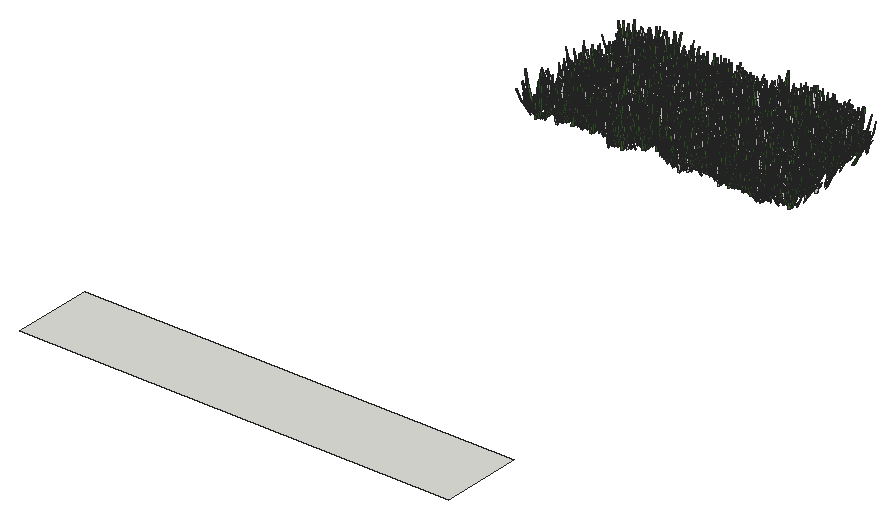
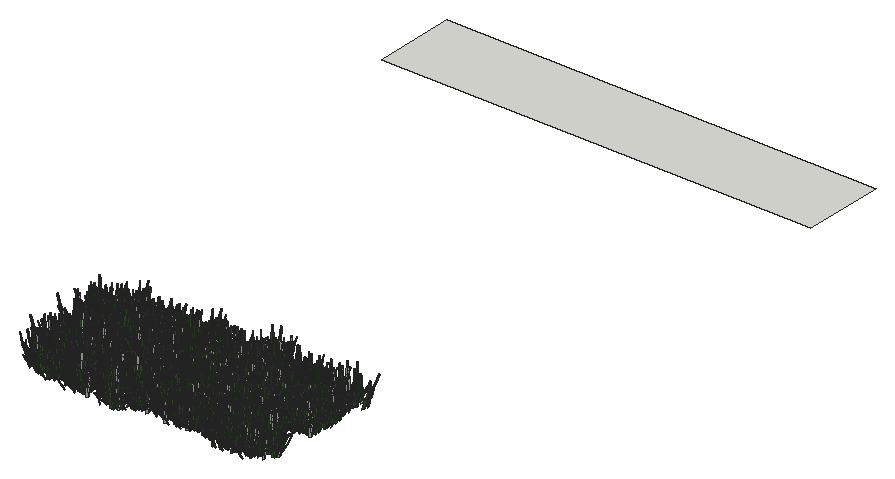
# SketchUp Ruby script. Lengths in inches.
U = 1.inch
M = Sketchup.active_model
def pt(a) = Geom::Point3d.new(a.map { |v| v * U })
def face(e, loops, mat)
  f = e.add_face(loops[0].map { |a| pt(a) })
  loops[1..].each { |l| e.add_face(l.map { |a| pt(a) }).erase! }
  f.material = f.back_material = mat if mat
  f
end
# faces: each face lists its corners as indices into pts; further lists are holes
def faces(e, pts, list, mat = nil) = list.each { |f| face(e, (f[0].is_a?(Array) ? f : [f]).map { |l| l.map { |i| pts[i] } }, mat) }
# xy, xz, yz: faces in a plane at the given z, y or x. An outline is a flat list of corners, or four numbers for a rectangle; further outlines are holes
def ring(l) = l.size == 4 ? [[l[0], l[1]], [l[2], l[1]], [l[2], l[3]], [l[0], l[3]]] : l.each_slice(2).to_a
def flat(e, list, mat, &to3) = list.each { |f| face(e, (f[0].is_a?(Array) ? f : [f]).map { |l| ring(l).map { |u, v| to3.(u, v) } }, mat) }
def xy(e, z, list, mat = nil) = flat(e, list, mat) { |x, y| [x, y, z] }
def xz(e, y, list, mat = nil) = flat(e, list, mat) { |x, z| [x, y, z] }
def yz(e, x, list, mat = nil) = flat(e, list, mat) { |y, z| [x, y, z] }
def lines(e, pts, list) = list.each { |a, b| e.add_line(pt(pts[a]), pt(pts[b])) }
# prism: a flat outline (further loops are holes) pulled along v
def prism(e, loops, v, mat = nil)
  f = face(e, loops, mat); d = Geom::Vector3d.new(v.map { |x| x * U })
  f.pushpull(f.normal.samedirection?(d) ? d.length : -d.length)
end
def box(e, o, s, mat = nil) = prism(e, [[o, [o[0] + s[0], o[1], o[2]], [o[0] + s[0], o[1] + s[1], o[2]], [o[0], o[1] + s[1], o[2]]]], [0, 0, s[2]], mat)
def at(x, y, z, deg = 0) = Geom::Transformation.translation(pt([x, y, z])) * Geom::Transformation.rotation(ORIGIN, Z_AXIS, deg.degrees)
def axes(o, x, y, z) = Geom::Transformation.new([*x, 0, *y, 0, *z, 0, *pt(o).to_a, 1])
def part(name) = M.definitions.add(name)
# library, detail: a bought-in or finely detailed component or shape, given as its bounding box
def library(name, o, s) = part(name).tap { |d| box(d.entities, o, s) }
def detail(e, o, s) = box(e.add_group.entities, o, s)
def put(e, d, t, mat = nil) = e.add_instance(d, t).tap { |i| i.material = mat if mat }
def group(e, t, mat = nil) = e.add_group.tap { |g| g.transformation = t; g.material = mat if mat }.entities
root = M.entities
M.materials.add("Material1").color = [58, 110, 58]
M.materials.add("Material10").color = [48, 100, 38]
M.materials.add("Material3").color = [68, 110, 58]
M.materials.add("Material4").color = [48, 90, 38]
M.materials.add("Material5").color = [68, 110, 48]
M.materials.add("Material6").color = [48, 90, 48]
M.materials.add("Material8").color = [58, 90, 38]
M.materials.add("Material9").color = [68, 100, 58]
c1 = part("grass00")
p = [[-0.6875,0.15,0],[-0.56,0.08,5.52],[-0.04,0.03,2.76],[0.48,-0.02,0],[0.35,-0.02,5.52],[-0.1,-0.14,5.52],
  [-0.12,0.65,8.37],[-0.42,0.65,8.37]]
faces(c1.entities,p,[[0,1,2,3],[3,2,4],[1,5,2],[5,4,2],[1,6,5],[4,5,6],[7,6,1]])
c2 = part("Group16\#1")
put(c2.entities,c1,axes([1.44,-0.61,-0.01],[0.05352,0.12609,0],[-0.10704,0.04543,0.07239],[0.06664,-0.02828,0.11628]),"Material6")
put(c2.entities,c1,axes([0.76,-0.15,-0.01],[0.04676,0.24062,0],[-0.23162,0.04501,0.06642],[0.0652,-0.01267,0.23595]),"Material3")
put(c2.entities,c1,axes([0.79,0.01,-0.01],[-0.00606,0.34651,0],[-0.34381,-0.00602,0.0432],[0.04319,0.00076,0.34386]))
put(c2.entities,c1,axes([1,0.23,-0.01],[-0.07192,0.31144,0],[-0.28722,-0.06632,0.1236],[0.12043,0.02781,0.29478]),"Material5")
put(c2.entities,c1,axes([1.66,0.77,-0.01],[-0.13828,0.29651,0],[-0.21551,-0.1005,0.22471],[0.20365,0.09498,0.23779]),"Material10")
put(c2.entities,c1,axes([0.6875,0.52,-0.01],[-0.18126,0.24051,0],[-0.22746,-0.17142,0.09788],[0.07817,0.05891,0.28481]),"Material5")
put(c2.entities,c1,axes([0.68,0.78,-0.01],[-0.215,0.18688,0],[-0.12385,-0.14248,0.21334],[0.13995,0.16101,0.18878]),"Material3")
put(c2.entities,c1,axes([0.56,1,-0.01],[-0.13756,0.07624,0],[-0.06159,-0.11112,0.0927],[0.04494,0.08108,0.12705]),"Material5")
put(c2.entities,c1,axes([0.2,0.64,-0.01],[-0.23729,0.07254,0],[-0.05711,-0.18681,0.153],[0.04473,0.14632,0.19535]),"Material10")
put(c2.entities,c1,axes([0.0625,0.72,-0.01],[-0.28874,0.02525,0],[-0.02179,-0.24916,0.14647],[0.01276,0.14591,0.25012]),"Material3")
put(c2.entities,c1,axes([-0.08,0.62,-0.01],[-0.34089,-0.04187,0],[0.03255,-0.26504,0.216],[-0.02633,0.21439,0.26703]),"Material10")
put(c2.entities,c1,axes([-0.34,0.98,-0.01],[-0.14314,-0.0493,0],[0.04397,-0.12769,0.06843],[-0.02228,0.0647,0.13505]),"Material10")
put(c2.entities,c1,axes([-0.87,1.45,-0.01],[-0.23488,-0.14114,0],[0.13761,-0.22901,0.06087],[-0.03135,0.05217,0.26717]))
put(c2.entities,c1,axes([-0.72,0.77,-0.01],[-0.14208,-0.13251,0],[0.07209,-0.0773,0.16301],[-0.11118,0.11922,0.1057]),"Material10")
put(c2.entities,c1,axes([-0.62,0.43,-0.01],[-0.14845,-0.21203,0],[0.18654,-0.13061,0.12304],[-0.10079,0.07057,0.22772]),"Material3")
put(c2.entities,c1,axes([-0.68,0.29,-0.01],[-0.13639,-0.32136,0],[0.31723,-0.13464,0.05579],[-0.05136,0.0218,0.34462]),"Material4")
put(c2.entities,c1,axes([-0.64,0.125,-0.01],[-0.0458,-0.23569,0],[0.22124,-0.043,0.08276],[-0.08124,0.01579,0.22538]),"Material1")
put(c2.entities,c1,axes([-1.6,-0.03,-0.01],[0.00576,-0.32897,0],[0.27526,0.00482,0.18018],[-0.18015,-0.00315,0.2753]),"Material5")
put(c2.entities,c1,axes([-1.36,-0.31,-0.01],[0.05718,-0.24765,0],[0.18172,0.04196,0.17267],[-0.16825,-0.03885,0.1865]),"Material10")
put(c2.entities,c1,axes([-1.54,-0.72,-0.01],[0.06537,-0.14017,0],[0.13555,0.06321,0.03939],[-0.0357,-0.01665,0.14956]))
put(c2.entities,c1,axes([-1.19,-0.9,-0.01],[0.09597,-0.12735,0],[0.11214,0.08451,0.07557],[-0.06035,-0.04548,0.14042]),"Material9")
put(c2.entities,c1,axes([-0.47,-0.54,-0.01],[0.11588,-0.10072,0],[0.0618,0.0711,0.12124],[-0.07953,-0.0915,0.0942]))
put(c2.entities,c1,axes([-0.47,-0.84,-0.01],[0.11927,-0.0661,0],[0.06603,0.11913,0.00646],[-0.00313,-0.00565,0.13621]),"Material5")
put(c2.entities,c1,axes([-0.38,-1.24,-0.01],[0.28037,-0.08571,0],[0.0618,0.20215,0.20315],[-0.05939,-0.19428,0.21139]),"Material9")
put(c2.entities,c1,axes([-0.06,-0.66,-0.01],[0.22719,-0.01987,0],[0.01247,0.14255,0.17758],[-0.01547,-0.17691,0.1431]),"Material8")
put(c2.entities,c1,axes([0.11,-0.89,-0.01],[0.14882,0.01828,0],[-0.01058,0.08611,0.12229],[0.01491,-0.12138,0.08676]),"Material6")
put(c2.entities,c1,axes([0.25,-0.72,-0.01],[0.20481,0.07053,0],[-0.06206,0.18022,0.10291],[0.03351,-0.0973,0.1906]),"Material6")
put(c2.entities,c1,axes([0.85,-1.42,-0.01],[0.16481,0.09904,0],[-0.09472,0.15762,0.05616],[0.02893,-0.04814,0.18389]),"Material5")
put(c2.entities,c1,axes([1.01,-1.09,-0.01],[0.21858,0.20385,0],[-0.17495,0.1876,0.15339],[0.10462,-0.11218,0.25652]),"Material10")
put(c2.entities,c1,axes([1.01,-0.71,-0.01],[0.08733,0.12473,0],[-0.06445,0.04512,0.13037],[0.1068,-0.07477,0.07867]),"Material6")
c3 = part("Group15\#1")
put(c3.entities,c2,at(0,0,0))
c4 = part("3darcstudiotree_grass00\#1")
put(c4.entities,c3,at(0,0,0))
xy(root,0,[[282.38,19.38,346,31.39]])
put(root,c4,axes([297.61,97.11,0.25],[1.11442,-0.27325,0],[0.34617,0.97258,-0.05518],[0.02268,0.06373,1.77288]))
put(root,c4,axes([309.04,97.14,0.25],[-0.81622,0.63511,0],[-0.72135,-0.63864,-0.04557],[-0.05793,-0.05129,1.96028]))
put(root,c4,axes([318.15,97.38,0.25],[-0.95081,0.11233,0],[-0.13919,-0.81164,-0.03826],[-0.00903,-0.05267,1.65468]))
put(root,c4,axes([324.87,97.82,0.25],[0.99592,-0.02661,0],[0.02899,0.74764,-0.04101],[0.00201,0.05178,1.37186]))
put(root,c4,axes([326.48,98.03,0.25],[1.16611,0.10212,0],[-0.10117,0.79586,-0.03171],[-0.00592,0.04657,1.71518]))
put(root,c4,axes([330.21,97.79,0.25],[0.11865,0.89123,0],[-0.92054,0.08443,-0.03685],[-0.06873,0.0063,1.73767]))
put(root,c4,axes([304.1,98.11,0.25],[1.12096,0.07204,0],[-0.08662,0.92856,-0.0417],[-0.00549,0.05888,1.91485]))
put(root,c4,axes([324.01,97.96,0.25],[-0.93317,0.25697,0],[-0.32463,-0.81214,-0.04681],[-0.02202,-0.05508,1.53984]))
put(root,c4,axes([300.77,97.91,0.25],[-0.99958,0.5509,0],[-0.69845,-0.87305,-0.05111],[-0.03443,-0.04304,1.53759]))
put(root,c4,axes([308.39,98.12,0.25],[-0.94502,0.15563,0],[-0.24855,-1.03972,-0.05548],[-0.01391,-0.05818,1.6451]))
put(root,c4,axes([302.0625,98.48,0.25],[0.91722,-0.25224,0],[0.3035,0.7603,-0.03222],[0.01878,0.04704,1.78787]))
put(root,c4,axes([332.7,98.4375,0.25],[1.19981,0.30777,0],[-0.3695,0.99233,-0.04987],[-0.01901,0.05104,1.61513]))
put(root,c4,axes([328.71,98.2,0.25],[-0.13885,0.83735,0],[-1.13883,-0.13009,-0.0385],[-0.05163,-0.0059,1.55608]))
put(root,c4,axes([318.98,98.26,0.25],[0.07462,0.91972,0],[-0.97751,0.05464,-0.04154],[-0.07881,0.00441,1.86323]))
put(root,c4,axes([315.89,98.68,0.25],[0.09651,-0.80548,0],[0.96144,0.07936,-0.03727],[0.06649,0.00549,1.73202]))
put(root,c4,axes([321.23,98.59,0.25],[-0.42768,-0.67094,0],[0.95175,-0.41794,-0.0302],[0.04153,-0.01824,1.67548]))
put(root,c4,axes([311.67,98.66,0.25],[0.80756,0.80599,0],[-0.89495,0.61773,-0.02991],[-0.03862,0.02666,1.95467]))
put(root,c4,axes([322.41,99.12,0.25],[0.43279,-0.82555,0],[1.00075,0.36142,-0.04597],[0.05367,0.01938,1.38947]))
put(root,c4,axes([328.51,99.08,0.25],[-0.59328,0.73911,0],[-0.83118,-0.45962,-0.03773],[-0.04449,-0.0246,1.41517]))
put(root,c4,axes([299.35,99.12,0.25],[-0.22047,0.82927,0],[-1.14406,-0.20954,-0.05256],[-0.05732,-0.0105,1.30827]))
put(root,c4,axes([308.98,99.51,0.25],[0.31203,-0.81509,0],[1.23306,0.32518,-0.03698],[0.04985,0.01315,1.82987]))
put(root,c4,axes([317.5,99.3,0.25],[-1.00537,-0.3617,0],[0.36325,-0.69557,-0.04544],[0.0295,-0.05648,1.4908]))
put(root,c4,axes([304.08,99.45,0.25],[0.99013,0.44406,0],[-0.59296,0.91082,-0.05913],[-0.03144,0.0483,1.39517]))
put(root,c4,axes([324.36,99.86,0.25],[-0.68424,-0.62612,0],[0.77326,-0.58215,-0.0539],[0.05475,-0.04122,1.43163]))
put(root,c4,axes([312.68,99.88,0.25],[0.97858,0.24585,0],[-0.28536,0.7825,-0.0422],[-0.02332,0.06396,1.87907]))
put(root,c4,axes([301.36,99.81,0.25],[0.11207,0.80416,0],[-0.996,0.09562,-0.04522],[-0.0721,0.00692,1.60941]))
put(root,c4,axes([330.24,99.96,0.25],[-0.79621,-0.4404,0],[0.66053,-0.82267,-0.04785],[0.04066,-0.05064,1.82518]))
put(root,c4,axes([298.22,100.3125,0.25],[0.22875,-0.9605,0],[1.22208,0.2005,-0.04547],[0.0618,0.01014,1.72572]))
put(root,c4,axes([320.22,100.33,0.25],[1.29123,-0.11334,0],[0.13389,1.05087,-0.02611],[0.00423,0.03321,1.96192]))
put(root,c4,axes([313.45,100.29,0.25],[-0.17956,-0.84679,0],[1.25977,-0.18403,-0.05842],[0.08919,-0.01303,1.98292]))
put(root,c4,axes([302.2,100.43,0.25],[0.02759,0.77056,0],[-1.10892,0.02736,-0.05613],[-0.07716,0.0019,1.5259]))
put(root,c4,axes([331.22,100.58,0.25],[-0.75484,-0.55993,0],[0.64882,-0.60256,-0.04195],[0.04472,-0.04153,1.55746]))
put(root,c4,axes([318.8,100.71,0.25],[1.03911,0.09401,0],[-0.10137,0.77188,-0.03498],[-0.00601,0.0458,1.48455]))
put(root,c4,axes([324.91,100.49,0.25],[-0.85951,0.28596,0],[-0.412,-0.8531,-0.04281],[-0.0261,-0.05404,1.81418]))
put(root,c4,axes([314.73,100.51,0.25],[-0.22146,0.9116,0],[-1.23324,-0.20639,-0.03197],[-0.04449,-0.00745,1.78572]))
put(root,c4,axes([328.82,100.9,0.25],[1.17011,-0.34767,0],[0.39668,0.91972,-0.05713],[0.02422,0.05616,1.48067]))
put(root,c4,axes([311.82,100.56,0.25],[-0.5993,0.62128,0],[-0.79962,-0.53137,-0.02462],[-0.03671,-0.02439,1.95656]))
put(root,c4,axes([307.43,100.74,0.25],[0.05722,0.94648,0],[-1.16997,0.04872,-0.03261],[-0.05169,0.00215,1.85888]))
put(root,c4,axes([332.53,100.92,0.25],[-0.75241,-0.52207,0],[0.686,-0.6811,-0.04185],[0.04373,-0.04342,1.7425]))
put(root,c4,axes([304.37,100.9,0.25],[-1.04972,-0.29462,0],[0.37971,-0.93199,-0.06149],[0.02998,-0.07358,1.80385]))
put(root,c4,axes([310.51,101.17,0.25],[0.10575,-0.82311,0],[0.95887,0.08487,-0.04937],[0.08765,0.00776,1.72169]))
put(root,c4,axes([317.53,101.08,0.25],[0.831,0.29847,0],[-0.361,0.69242,-0.02703],[-0.02268,0.04351,1.9211]))
put(root,c4,axes([299.71,100.85,0.25],[-0.333,0.90097,0],[-0.9209,-0.23448,-0.03727],[-0.05842,-0.01487,1.57911]))
put(root,c4,axes([322.65,101.03,0.25],[-1.17026,-0.36941,0],[0.34854,-0.76064,-0.04106],[0.0256,-0.05587,1.71966]))
put(root,c4,axes([305.88,100.9,0.25],[-0.57732,0.57346,0],[-0.80073,-0.55534,-0.03387],[-0.03843,-0.02665,1.54303]))
put(root,c4,axes([309.86,101.96,0.25],[1.05783,0.04505,0],[-0.06563,1.06167,-0.05168],[-0.00349,0.05647,1.68853]))
put(root,c4,axes([297.7,101.96,0.25],[-0.14741,-0.93143,0],[0.95379,-0.10399,-0.04534],[0.07585,-0.00827,1.62314]))
put(root,c4,axes([323.3125,101.95,0.25],[-0.30211,-0.82943,0],[1.20998,-0.30361,-0.03772],[0.03909,-0.00981,1.36861]))
put(root,c4,axes([305.84,102.15,0.25],[0.91341,-0.33571,0],[0.50825,0.95265,-0.04981],[0.02823,0.05291,1.75709]))
put(root,c4,axes([326.74,101.86,0.25],[-1.11386,0.29268,0],[-0.32243,-0.84536,-0.03323],[-0.01665,-0.04365,1.77353]))
put(root,c4,axes([330.87,102.33,0.25],[1.03086,-0.47818,0],[0.57832,0.85889,-0.04605],[0.0263,0.03906,1.38783]))
put(root,c4,axes([315.96,101.99,0.25],[-0.9413,0.11811,0],[-0.18993,-1.04277,-0.03474],[-0.00584,-0.03204,1.42794]))
put(root,c4,axes([299.58,102.47,0.25],[0.63325,-0.82651,0],[0.82121,0.43345,-0.04064],[0.05169,0.02728,1.46692]))
put(root,c4,axes([329.73,102.18,0.25],[-0.64705,0.66274,0],[-0.92031,-0.61899,-0.04128],[-0.04141,-0.02785,1.52936]))
put(root,c4,axes([321.76,102.83,0.25],[1.05012,0.46296,0],[-0.47019,0.73472,-0.04207],[-0.03729,0.05828,1.89419]))
put(root,c4,axes([317.68,102.97,0.25],[-0.58739,0.78346,0],[-1.04255,-0.53848,-0.04897],[-0.06631,-0.03425,1.9584]))
put(root,c4,axes([316.28,103.14,0.25],[0.67846,0.67759,0],[-0.85974,0.59303,-0.05468],[-0.0598,0.04125,1.58958]))
put(root,c4,axes([306.8,103.52,0.25],[0.95094,-0.43354,0],[0.56411,0.8524,-0.02691],[0.01977,0.02987,1.78778]))
put(root,c4,axes([297.72,103.32,0.25],[-0.9964,-0.33803,0],[0.35737,-0.72569,-0.04864],[0.0279,-0.05665,1.4319]))
put(root,c4,axes([332.73,103.31,0.25],[-1.12743,-0.30714,0],[0.33973,-0.85911,-0.0393],[0.01924,-0.04865,1.71017]))
put(root,c4,axes([320.33,103.1875,0.25],[-0.89951,0.48737,0],[-0.66735,-0.8485,-0.04574],[-0.03789,-0.04818,1.85022]))
put(root,c4,axes([305.19,103.68,0.25],[0.59611,-0.65972,0],[0.97376,0.60614,-0.03529],[0.03147,0.01959,1.35654]))
put(root,c4,axes([310.63,103.33,0.25],[0.11273,0.93049,0],[-0.9606,0.08017,-0.04963],[-0.07565,0.00631,1.47912]))
put(root,c4,axes([326.61,104.0625,0.25],[-0.46457,-0.99645,0],[1.15948,-0.3724,-0.05475],[0.07745,-0.02488,1.88574]))
put(root,c4,axes([312.78,104.58,0.25],[0.42125,-0.83748,0],[1.16384,0.40329,-0.03949],[0.05184,0.01796,1.7941]))
put(root,c4,axes([328.78,104.7,0.25],[0.63809,-0.69669,0],[1.02647,0.64766,-0.05929],[0.05496,0.03468,1.50135]))
put(root,c4,axes([325.85,104.61,0.25],[-0.57071,-0.88679,0],[1.05327,-0.46697,-0.05822],[0.083,-0.0368,1.92982]))
put(root,c4,axes([329.61,104.72,0.25],[1.1093,0.03312,0],[-0.04015,0.92644,-0.02702],[-0.00174,0.04004,1.99535]))
put(root,c4,axes([310.17,104.7,0.25],[-0.85657,-0.75846,0],[0.78932,-0.61411,-0.03051],[0.03395,-0.02642,1.65027]))
put(root,c4,axes([320.77,104.93,0.25],[-0.86,-0.30499,0],[0.49403,-0.95969,-0.04539],[0.0273,-0.05303,1.92461]))
put(root,c4,axes([298.375,104.8125,0.25],[-0.66373,0.7804,0],[-0.8847,-0.51835,-0.04566],[-0.05684,-0.03331,1.65042]))
put(root,c4,axes([307.43,104.95,0.25],[-0.81395,0.35466,0],[-0.55874,-0.88338,-0.02543],[-0.01877,-0.02968,1.9093]))
put(root,c4,axes([325.57,105.72,0.25],[1.07758,0.21503,0],[-0.30245,1.04413,-0.03506],[-0.00839,0.02898,1.32515]))
put(root,c4,axes([297.92,105.64,0.25],[0.96578,0.31729,0],[-0.34767,0.72902,-0.04887],[-0.03524,0.07388,1.85053]))
put(root,c4,axes([300.12,106.1,0.25],[0.88355,-0.55441,0],[0.65814,0.72256,-0.04167],[0.04286,0.04705,1.86151]))
put(root,c4,axes([312.65,106.09,0.25],[0.37476,-0.82487,0],[1.09143,0.3416,-0.04892],[0.07598,0.02378,1.93615]))
put(root,c4,axes([311.34,105.75,0.25],[-1.08648,0.48141,0],[-0.55382,-0.86106,-0.03463],[-0.0258,-0.04011,1.86049]))
put(root,c4,axes([301.49,105.85,0.25],[0.38225,0.93797,0],[-0.99384,0.27902,-0.04556],[-0.06331,0.01777,1.53888]))
put(root,c4,axes([305.43,105.83,0.25],[-1.09946,0.15846,0],[-0.20428,-0.97645,-0.05401],[-0.01022,-0.04885,1.3206]))
put(root,c4,axes([314.78,105.86,0.25],[-0.84958,0.7153,0],[-0.71377,-0.58402,-0.05097],[-0.06552,-0.05361,1.80901]))
put(root,c4,axes([323.95,106.21,0.25],[0.95429,0.31987,0],[-0.42632,0.8762,-0.03343],[-0.02074,0.04263,1.88641]))
put(root,c4,axes([307.34,106.1,0.25],[0.55377,0.81028,0],[-0.78931,0.37162,-0.03898],[-0.07426,0.03496,1.98748]))
put(root,c4,axes([322.34,106.65,0.25],[0.24209,-0.99141,0],[1.19956,0.20179,-0.041],[0.05797,0.00975,1.76588]))
put(root,c4,axes([314.92,106.6,0.25],[1.2191,0.02658,0],[-0.027,0.85312,-0.04419],[-0.00224,0.07077,1.98467]))
put(root,c4,axes([311.93,106.71,0.25],[-0.47441,-0.8123,0],[0.87704,-0.35287,-0.03263],[0.05634,-0.02267,1.87]))
put(root,c4,axes([320.57,107.07,0.25],[1.2067,-0.00105,0],[0.00128,1.01679,-0.04894],[0.00006,0.04681,1.41164]))
put(root,c4,axes([331.68,107.02,0.25],[0.99274,0.22293,0],[-0.25761,0.79027,-0.04799],[-0.02037,0.0625,1.60328]))
put(root,c4,axes([313.64,107.03,0.25],[-0.97842,-0.39566,0],[0.51576,-0.87863,-0.02869],[0.02026,-0.03451,1.89824]))
put(root,c4,axes([323.66,107.1,0.25],[0.80414,0.72555,0],[-0.85103,0.64979,-0.033],[-0.03942,0.0301,1.87715]))
put(root,c4,axes([303.6,107,0.25],[-0.75001,0.80323,0],[-1.01098,-0.65032,-0.03455],[-0.03376,-0.02172,1.58129]))
put(root,c4,axes([315.7,107.18,0.25],[-0.02112,0.92901,0],[-1.11715,-0.0175,-0.05443],[-0.07643,-0.0012,1.56933]))
put(root,c4,axes([327.87,107.3125,0.25],[-1.1857,0.2388,0],[-0.30456,-1.04174,-0.06662],[-0.01699,-0.0581,1.39642]))
put(root,c4,axes([310.27,107.51,0.25],[-0.87437,0.41705,0],[-0.6352,-0.91743,-0.04948],[-0.03099,-0.04476,1.60238]))
put(root,c4,axes([324.25,108.01,0.25],[-0.31424,-0.81036,0],[1.12057,-0.29935,-0.0477],[0.05342,-0.01427,1.385]))
put(root,c4,axes([318.85,107.99,0.25],[-1.13196,0.07822,0],[-0.0777,-0.77461,-0.02559],[-0.00443,-0.04414,1.95328]))
put(root,c4,axes([317.96,107.96,0.25],[-0.77412,0.64338,0],[-0.79625,-0.65999,-0.05526],[-0.05902,-0.04892,1.69871]))
put(root,c4,axes([314.45,108.38,0.25],[-0.14115,-0.84151,0],[1.08164,-0.12498,-0.04493],[0.07806,-0.00902,1.91565]))
put(root,c4,axes([325.47,108.53,0.25],[0.45572,-0.66105,0],[0.90705,0.43077,-0.04415],[0.07294,0.03464,1.98924]))
put(root,c4,axes([327.2,108.64,0.25],[1.09438,-0.24928,0],[0.33452,1.01172,-0.05143],[0.01553,0.04697,1.44218]))
put(root,c4,axes([328.73,108.71,0.25],[0.53158,-0.96832,0],[1.00993,0.38194,-0.02827],[0.04498,0.01701,1.94019]))
put(root,c4,axes([321.96,108.36,0.25],[0.25266,1.02917,0],[-1.10373,0.18666,-0.0503],[-0.06889,0.01165,1.57458]))
put(root,c4,axes([308.34,108.53,0.25],[-1.09634,-0.4052,0],[0.42135,-0.78536,-0.04343],[0.02306,-0.04299,1.35201]))
put(root,c4,axes([331.02,108.6,0.25],[0.75404,0.74158,0],[-0.73552,0.51522,-0.05003],[-0.07249,0.05078,1.82479]))
put(root,c4,axes([300.56,108.72,0.25],[-1.0242,0.40671,0],[-0.52839,-0.91667,-0.05113],[-0.02415,-0.04189,1.33965]))
put(root,c4,axes([316.64,109.125,0.25],[-0.04985,-0.8677,0],[1.12073,-0.04435,-0.05646],[0.07894,-0.00312,1.57058]))
put(root,c4,axes([313.23,109.14,0.25],[1.20436,-0.01732,0],[0.01668,0.79893,-0.04649],[0.00132,0.06305,1.57333]))
put(root,c4,axes([308.19,109.3,0.25],[0.58157,-0.91412,0],[0.81672,0.35796,-0.03491],[0.05523,0.02421,1.65255]))
put(root,c4,axes([306.07,109.5,0.25],[0.77973,-0.78258,0],[0.76132,0.52256,-0.04304],[0.05909,0.04056,1.76026]))
put(root,c4,axes([330.37,109.54,0.25],[1.0238,-0.14482,0],[0.16099,0.78402,-0.03176],[0.01034,0.05035,1.85682]))
put(root,c4,axes([325.35,109.36,0.25],[0.69121,0.91353,0],[-0.96464,0.50281,-0.052],[-0.06865,0.03579,1.7759]))
put(root,c4,axes([309.76,109.52,0.25],[0.40329,0.8772,0],[-0.97312,0.30821,-0.03212],[-0.04988,0.0158,1.73128]))
put(root,c4,axes([314.22,109.71,0.25],[-1.14349,-0.47242,0],[0.56245,-0.93786,-0.0574],[0.02865,-0.04778,1.41402]))
put(root,c4,axes([322.65,109.99,0.25],[1.07915,-0.5991,0],[0.50648,0.62849,-0.03191],[0.03494,0.04336,1.79443]))
put(root,c4,axes([319.76,109.71,0.25],[-0.53398,0.84817,0],[-1.13911,-0.49404,-0.06253],[-0.0818,-0.03548,1.89715]))
put(root,c4,axes([304.45,109.98,0.25],[-0.22919,0.77931,0],[-0.9756,-0.19765,-0.03757],[-0.04783,-0.00969,1.3158]))
put(root,c4,axes([331.35,110.47,0.25],[0.99421,-0.54602,0],[0.59381,0.74486,-0.03005],[0.02904,0.03643,1.88475]))
put(root,c4,axes([322.6,110.53,0.25],[0.65031,-0.90821,0],[0.82995,0.4094,-0.0411],[0.05579,0.02752,1.52451]))
put(root,c4,axes([315.1,110.54,0.25],[0.48323,-0.72234,0],[0.9231,0.42542,-0.03203],[0.04697,0.02165,1.771]))
put(root,c4,axes([313.6,110.58,0.25],[-1.02369,-0.45629,0],[0.46842,-0.72398,-0.0264],[0.02496,-0.03858,1.979]))
put(root,c4,axes([301.47,110.87,0.25],[-0.35269,-1.00211,0],[0.94351,-0.22876,-0.03009],[0.05064,-0.01228,1.72353]))
put(root,c4,axes([309.08,110.9375,0.25],[1.27878,-0.06749,0],[0.06526,0.85189,-0.03177],[0.00374,0.04884,1.90853]))
put(root,c4,axes([310.57,110.64,0.25],[-0.44299,0.8765,0],[-0.99668,-0.34702,-0.04701],[-0.07376,-0.02568,1.83905]))
put(root,c4,axes([312.18,110.99,0.25],[0.00713,-0.80021,0],[1.27202,0.00781,-0.04606],[0.06556,0.0004,1.81052]))
put(root,c4,axes([321.18,111.11,0.25],[0.73044,-0.43902,0],[0.61551,0.70549,-0.04376],[0.0427,0.04894,1.7457]))
put(root,c4,axes([304.66,111.28,0.25],[0.84421,-0.34427,0],[0.50716,0.85674,-0.05746],[0.04355,0.07356,1.97658]))
put(root,c4,axes([298.01,111.75,0.25],[0.68613,-0.76199,0],[0.80493,0.49931,-0.03861],[0.05418,0.03361,1.76068]))
put(root,c4,axes([314.57,111.68,0.25],[0.9074,0.55884,0],[-0.63165,0.70655,-0.02502],[-0.02679,0.02997,1.90511]))
put(root,c4,axes([315.76,111.9,0.25],[0.45912,-0.89515,0],[1.17392,0.41479,-0.03539],[0.03872,0.01368,1.51703]))
put(root,c4,axes([330.01,111.88,0.25],[1.04861,0.10322,0],[-0.13658,0.95588,-0.05841],[-0.00773,0.05413,1.30397]))
put(root,c4,axes([303.07,111.72,0.25],[0.42047,0.86427,0],[-1.07787,0.36125,-0.05886],[-0.06289,0.02108,1.33951]))
put(root,c4,axes([308.875,111.65,0.25],[-1.03901,0.52543,0],[-0.58281,-0.79394,-0.05764],[-0.04826,-0.06574,1.8024]))
put(root,c4,axes([299.62,112.18,0.25],[1.17343,-0.25453,0],[0.24845,0.78906,-0.02428],[0.01246,0.03956,1.99391]))
put(root,c4,axes([331.07,112.17,0.25],[0.64832,0.78454,0],[-0.80982,0.46102,-0.03781],[-0.05547,0.03158,1.74723]))
put(root,c4,axes([328.54,112.1,0.25],[0.20654,0.98643,0],[-0.89422,0.12898,-0.03272],[-0.06554,0.00945,1.8454]))
put(root,c4,axes([312.79,112.89,0.25],[1.24424,-0.04401,0],[0.04877,0.94984,-0.04096],[0.00262,0.05105,1.72127]))
put(root,c4,axes([305.8,112.99,0.25],[-0.18898,-0.77762,0],[1.1445,-0.19161,-0.04603],[0.06408,-0.01073,1.65834]))
put(root,c4,axes([308.18,113,0.25],[1.08717,0.39304,0],[-0.42636,0.81245,-0.04191],[-0.02079,0.03962,1.32656]))
put(root,c4,axes([331.11,112.89,0.25],[0.28621,0.85359,0],[-1.17682,0.27183,-0.02844],[-0.04085,0.00943,1.82107]))
put(root,c4,axes([304.47,112.92,0.25],[-1.08813,0.33223,0],[-0.34755,-0.7842,-0.04924],[-0.03349,-0.07558,1.98345]))
put(root,c4,axes([323.74,113.125,0.25],[-0.8674,-0.38833,0],[0.4459,-0.68613,-0.04409],[0.03307,-0.05089,1.48398]))
put(root,c4,axes([310.21,113.23,0.25],[0.88682,0.36393,0],[-0.44195,0.74191,-0.03066],[-0.02386,0.04005,1.75054]))
put(root,c4,axes([316.6,113.3,0.25],[0.83678,0.55471,0],[-0.6975,0.72485,-0.04015],[-0.03132,0.03255,1.39698]))
put(root,c4,axes([329.61,113.12,0.25],[-0.07913,1.00018,0],[-0.91633,-0.04994,-0.03425],[-0.06011,-0.00328,1.61497]))
put(root,c4,axes([320.41,113.28,0.25],[-1.01674,-0.27605,0],[0.2905,-0.7371,-0.035],[0.02017,-0.05118,1.73222]))
put(root,c4,axes([328.47,113.39,0.25],[0.80749,0.55955,0],[-0.76405,0.75959,-0.05497],[-0.05229,0.05198,1.76958]))
put(root,c4,axes([300.76,113.35,0.25],[-0.5872,0.68156,0],[-0.92382,-0.54831,-0.05929],[-0.06013,-0.03569,1.41608]))
put(root,c4,axes([325.14,113.4375,0.25],[-0.46766,0.64426,0],[-1.08655,-0.54335,-0.04504],[-0.05932,-0.02966,1.9506]))
put(root,c4,axes([299.41,113.71,0.25],[0.61607,0.69409,0],[-0.89384,0.54656,-0.0323],[-0.03504,0.02143,1.496]))
put(root,c4,axes([324.16,114.25,0.25],[1.24288,0.31106,0],[-0.29758,0.81912,-0.04516],[-0.02281,0.0628,1.80387]))
put(root,c4,axes([302.67,114.27,0.25],[-1.05804,-0.34038,0],[0.39783,-0.8519,-0.05586],[0.03523,-0.07545,1.92103]))
put(root,c4,axes([319.06,114.5,0.25],[0.27403,-0.76495,0],[1.21167,0.29902,-0.06029],[0.08173,0.02017,1.78762]))
